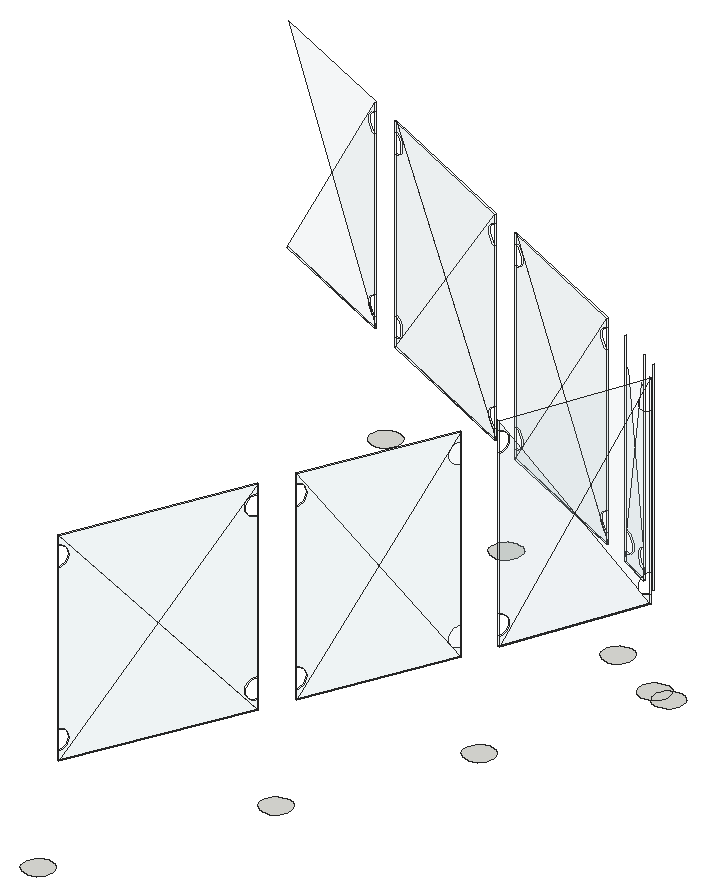
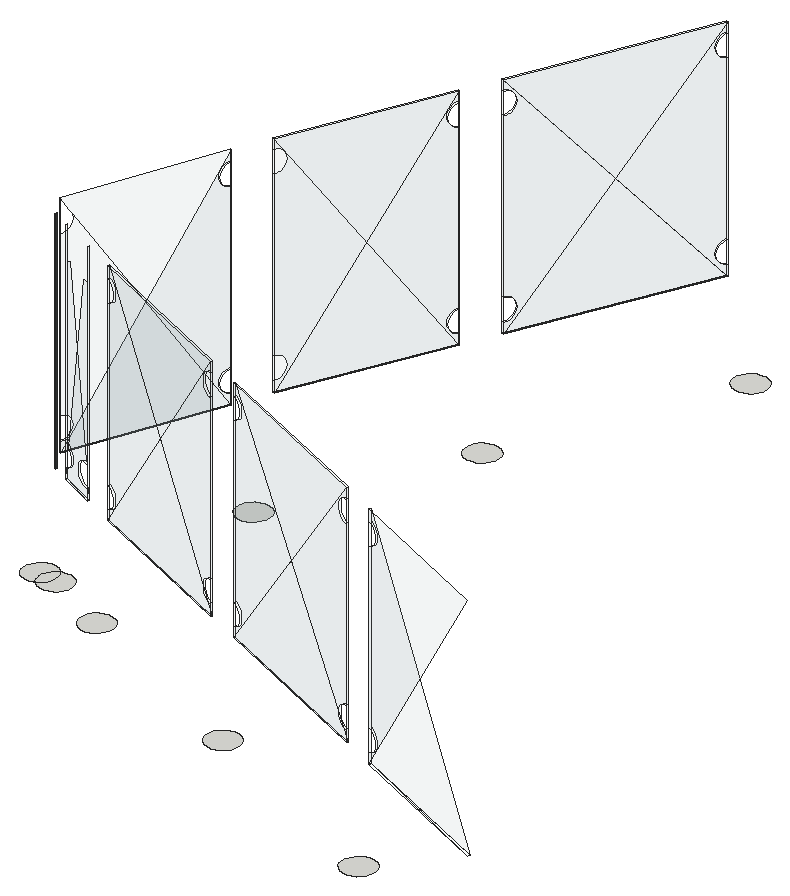
# SketchUp Ruby script. Lengths in inches.
U = 1.inch
M = Sketchup.active_model
def pt(a) = Geom::Point3d.new(a.map { |v| v * U })
def face(e, loops, mat)
  f = e.add_face(loops[0].map { |a| pt(a) })
  loops[1..].each { |l| e.add_face(l.map { |a| pt(a) }).erase! }
  f.material = f.back_material = mat if mat
  f
end
# faces: each face lists its corners as indices into pts; further lists are holes
def faces(e, pts, list, mat = nil) = list.each { |f| face(e, (f[0].is_a?(Array) ? f : [f]).map { |l| l.map { |i| pts[i] } }, mat) }
# xy, xz, yz: faces in a plane at the given z, y or x. An outline is a flat list of corners, or four numbers for a rectangle; further outlines are holes
def ring(l) = l.size == 4 ? [[l[0], l[1]], [l[2], l[1]], [l[2], l[3]], [l[0], l[3]]] : l.each_slice(2).to_a
def flat(e, list, mat, &to3) = list.each { |f| face(e, (f[0].is_a?(Array) ? f : [f]).map { |l| ring(l).map { |u, v| to3.(u, v) } }, mat) }
def xy(e, z, list, mat = nil) = flat(e, list, mat) { |x, y| [x, y, z] }
def xz(e, y, list, mat = nil) = flat(e, list, mat) { |x, z| [x, y, z] }
def yz(e, x, list, mat = nil) = flat(e, list, mat) { |y, z| [x, y, z] }
def lines(e, pts, list) = list.each { |a, b| e.add_line(pt(pts[a]), pt(pts[b])) }
# prism: a flat outline (further loops are holes) pulled along v
def prism(e, loops, v, mat = nil)
  f = face(e, loops, mat); d = Geom::Vector3d.new(v.map { |x| x * U })
  f.pushpull(f.normal.samedirection?(d) ? d.length : -d.length)
end
def box(e, o, s, mat = nil) = prism(e, [[o, [o[0] + s[0], o[1], o[2]], [o[0] + s[0], o[1] + s[1], o[2]], [o[0], o[1] + s[1], o[2]]]], [0, 0, s[2]], mat)
def at(x, y, z, deg = 0) = Geom::Transformation.translation(pt([x, y, z])) * Geom::Transformation.rotation(ORIGIN, Z_AXIS, deg.degrees)
def axes(o, x, y, z) = Geom::Transformation.new([*x, 0, *y, 0, *z, 0, *pt(o).to_a, 1])
def part(name) = M.definitions.add(name)
# library, detail: a bought-in or finely detailed component or shape, given as its bounding box
def library(name, o, s) = part(name).tap { |d| box(d.entities, o, s) }
def detail(e, o, s) = box(e.add_group.entities, o, s)
def put(e, d, t, mat = nil) = e.add_instance(d, t).tap { |i| i.material = mat if mat }
def group(e, t, mat = nil) = e.add_group.tap { |g| g.transformation = t; g.material = mat if mat }.entities
root = M.entities
M.materials.add("Glass_Safety_01").color = [204, 235, 244]
M.materials["Glass_Safety_01"].alpha = 0.1
xy(root,321.858,[[999.761,953.602,1000.164,953.685,1000.532,953.869,1000.839,954.142,1001.065,954.485,1001.195,954.875,1001.219,955.286,1001.137,955.688,1000.953,956.056,1000.68,956.363,1000.337,956.59,999.946,956.719,999.536,956.744,999.133,956.661,998.766,956.477,998.458,956.204,998.232,955.861,998.102,955.471,998.078,955.06,998.161,954.658,998.345,954.29,998.618,953.983,998.961,953.756,999.351,953.627],[1009.107,975.06,1009.51,975.143,1009.877,975.327,1010.185,975.6,1010.411,975.943,1010.541,976.333,1010.565,976.744,1010.482,977.146,1010.298,977.514,1010.025,977.821,1009.682,978.048,1009.292,978.177,1008.882,978.202,1008.479,978.119,1008.111,977.935,1007.804,977.662,1007.578,977.319,1007.448,976.929,1007.423,976.518,1007.506,976.116,1007.69,975.748,1007.963,975.441,1008.306,975.214,1008.696,975.085],[1017.079,993.365,1017.482,993.447,1017.849,993.631,1018.157,993.904,1018.383,994.248,1018.513,994.638,1018.537,995.048,1018.455,995.451,1018.27,995.818,1017.998,996.126,1017.654,996.352,1017.264,996.482,1016.854,996.506,1016.451,996.424,1016.084,996.24,1015.776,995.967,1015.55,995.623,1015.42,995.233,1015.396,994.823,1015.478,994.42,1015.662,994.053,1015.935,993.745,1016.279,993.519,1016.669,993.389],[1023.991,1011.073,1024.394,1011.156,1024.762,1011.34,1025.069,1011.613,1025.295,1011.956,1025.425,1012.346,1025.45,1012.756,1025.367,1013.159,1025.183,1013.527,1024.91,1013.834,1024.567,1014.061,1024.177,1014.19,1023.766,1014.215,1023.363,1014.132,1023.238,1014.069,1023.367,1013.924,1023.551,1013.556,1023.634,1013.153,1023.609,1012.743,1023.48,1012.353,1023.253,1012.01,1022.946,1011.737,1022.704,1011.616,1022.848,1011.454,1023.191,1011.227,1023.581,1011.098],[1022.175,1011.47,1022.578,1011.553,1022.704,1011.616,1022.575,1011.761,1022.391,1012.129,1022.308,1012.531,1022.332,1012.942,1022.462,1013.332,1022.688,1013.675,1022.996,1013.948,1023.238,1014.069,1023.094,1014.231,1022.751,1014.457,1022.361,1014.587,1021.95,1014.611,1021.548,1014.529,1021.18,1014.345,1020.873,1014.072,1020.646,1013.729,1020.516,1013.338,1020.492,1012.928,1020.575,1012.525,1020.759,1012.158,1021.032,1011.85,1021.375,1011.624,1021.765,1011.494],
  [1022.704,1011.616,1022.946,1011.737,1023.253,1012.01,1023.48,1012.353,1023.609,1012.743,1023.634,1013.153,1023.551,1013.556,1023.367,1013.924,1023.238,1014.069,1022.996,1013.948,1022.688,1013.675,1022.462,1013.332,1022.332,1012.942,1022.308,1012.531,1022.391,1012.129,1022.575,1011.761],[1015.608,1014.567,1016.011,1014.65,1016.378,1014.834,1016.686,1015.107,1016.912,1015.45,1017.042,1015.84,1017.066,1016.251,1016.983,1016.653,1016.799,1017.021,1016.526,1017.328,1016.183,1017.555,1015.793,1017.684,1015.383,1017.709,1014.98,1017.626,1014.612,1017.442,1014.305,1017.169,1014.079,1016.826,1013.949,1016.436,1013.924,1016.025,1014.007,1015.623,1014.191,1015.255,1014.464,1014.948,1014.807,1014.721,1015.197,1014.592],[996.475,1022.9,996.878,1022.983,997.246,1023.167,997.553,1023.44,997.779,1023.783,997.909,1024.173,997.934,1024.583,997.851,1024.986,997.667,1025.354,997.394,1025.661,997.051,1025.887,996.661,1026.017,996.25,1026.042,995.848,1025.959,995.48,1025.775,995.172,1025.502,994.946,1025.159,994.816,1024.769,994.792,1024.358,994.875,1023.955,995.059,1023.588,995.332,1023.28,995.675,1023.054,996.065,1022.924],[975.893,1031.864,976.296,1031.947,976.663,1032.131,976.971,1032.404,977.197,1032.747,977.327,1033.137,977.351,1033.548,977.269,1033.95,977.085,1034.318,976.812,1034.625,976.468,1034.852,976.078,1034.981,975.668,1035.006,975.265,1034.923,974.898,1034.739,974.59,1034.466,974.364,1034.123,974.234,1033.733,974.21,1033.322,974.292,1032.92,974.476,1032.552,974.749,1032.245,975.093,1032.018,975.483,1031.889]])
xy(root,331.897,[[1000.525,956.939,1000.344,957.017,1008.365,974.939],[1000.344,957.017,1008.184,975.017,1008.365,974.939],[1009.871,978.396,1009.69,978.475,1016.348,993.269],[1009.69,978.475,1016.168,993.348,1016.348,993.269],[1017.774,996.733,1017.591,996.805,1023.329,1010.964],
  [1017.591,996.805,1023.145,1011.036,1023.329,1010.964],[1021.935,1012.968,1021.928,1012.969,1021.97,1013.162],[1021.935,1012.968,1021.97,1013.162,1021.977,1013.16],[1020.24,1013.791,1016.751,1015.437,1016.835,1015.615],[1020.24,1013.791,1016.835,1015.615,1020.324,1013.969],
  [1013.651,1016.834,997.958,1023.669,998.037,1023.849],[1013.651,1016.834,998.037,1023.849,1013.73,1017.014],[994.519,1025.167,977.388,1032.628,977.466,1032.808],[994.519,1025.167,977.466,1032.808,994.597,1025.347],[973.936,1034.131,958.914,1040.674,958.992,1040.854],
  [973.936,1034.131,958.992,1040.854,974.015,1034.311]],"Glass_Safety_01")
p = [[1000.344,957.017,331.897],[1000.525,956.939,331.897],[1000.525,956.939,333],[1000.525,956.939,335.125],[1000.525,956.939,351.283],[1000.525,956.939,353.409],
  [1000.525,956.939,354.511],[1000.344,957.017,354.511],[1000.344,957.017,353.409],[1000.344,957.017,351.283],[1000.344,957.017,335.125],[1000.344,957.017,333],
  [1000.635,957.191,335.089],[1000.737,957.426,334.983],[1000.825,957.628,334.814],[1000.893,957.783,334.594],[1000.935,957.88,334.338],[1000.949,957.913,334.0625],
  [1000.935,957.88,333.787],[1000.893,957.783,333.531],[1000.825,957.628,333.311],[1000.737,957.426,333.142],[1000.635,957.191,333.036],[1008.365,974.939,354.511],
  [1000.635,957.191,353.373],[1000.737,957.426,353.267],[1000.825,957.628,353.098],[1000.893,957.783,352.877],[1000.935,957.88,352.621],[1000.949,957.913,352.346],
  [1000.935,957.88,352.071],[1000.893,957.783,351.814],[1000.825,957.628,351.594],[1000.737,957.426,351.425],[1000.635,957.191,351.319],[1008.365,974.939,331.897],
  [1008.365,974.939,333],[1008.298,974.787,333],[1008.189,974.535,333.036],[1008.086,974.3,333.142],[1007.998,974.098,333.311],[1007.931,973.943,333.531],
  [1007.888,973.846,333.787],[1007.874,973.8125,334.0625],[1007.888,973.846,334.338],[1007.931,973.943,334.594],[1007.998,974.098,334.814],[1008.086,974.3,334.983],
  [1008.189,974.535,335.089],[1008.298,974.787,335.125],[1008.365,974.939,335.125],[1008.365,974.939,351.283],[1008.298,974.787,351.283],[1008.189,974.535,351.319],
  [1008.086,974.3,351.425],[1007.998,974.098,351.594],[1007.931,973.943,351.814],[1007.888,973.846,352.071],[1007.874,973.8125,352.346],[1007.888,973.846,352.621],
  [1007.931,973.943,352.877],[1007.998,974.098,353.098],[1008.086,974.3,353.267],[1008.189,974.535,353.373],[1008.298,974.787,353.409],[1008.365,974.939,353.409],
  [1000.454,957.269,333.036],[1000.557,957.504,333.142],[1000.645,957.706,333.311],[1000.712,957.861,333.531],[1000.754,957.958,333.787],[1000.769,957.992,334.0625],
  [1000.754,957.958,334.338],[1000.712,957.861,334.594],[1000.645,957.706,334.814],[1000.557,957.504,334.983],[1000.454,957.269,335.089],[1000.454,957.269,351.319],
  [1000.557,957.504,351.425],[1000.645,957.706,351.594],[1000.712,957.861,351.814],[1000.754,957.958,352.071],[1000.769,957.992,352.346],[1000.754,957.958,352.621],
  [1000.712,957.861,352.877],[1000.645,957.706,353.098],[1000.557,957.504,353.267],[1000.454,957.269,353.373],[1008.184,975.017,331.897],[1008.184,975.017,351.283],
  [1008.184,975.017,335.125],[1008.118,974.865,335.125],[1008.008,974.613,335.089],[1007.906,974.378,334.983],[1007.818,974.176,334.814],[1007.75,974.021,334.594],
  [1007.708,973.924,334.338],[1007.694,973.891,334.0625],[1007.708,973.924,333.787],[1007.75,974.021,333.531],[1007.818,974.176,333.311],[1007.906,974.378,333.142],
  [1008.008,974.613,333.036],[1008.118,974.865,333],[1008.184,975.017,333],[1008.184,975.017,354.511],[1008.184,975.017,353.409],[1008.118,974.865,353.409],
  [1008.008,974.613,353.373],[1007.906,974.378,353.267],[1007.818,974.176,353.098],[1007.75,974.021,352.877],[1007.708,973.924,352.621],[1007.694,973.891,352.346],
  [1007.708,973.924,352.071],[1007.75,974.021,351.814],[1007.818,974.176,351.594],[1007.906,974.378,351.425],[1008.008,974.613,351.319],[1008.118,974.865,351.283],
  [1009.69,978.475,331.897],[1009.871,978.396,331.897],[1009.871,978.396,333],[1009.871,978.396,335.125],[1009.871,978.396,351.283],[1009.871,978.396,353.409],
  [1009.871,978.396,354.511],[1009.69,978.475,354.511],[1009.69,978.475,353.409],[1009.69,978.475,351.283],[1009.69,978.475,335.125],[1009.69,978.475,333],
  [1009.98,978.649,335.089],[1010.083,978.884,334.983],[1010.171,979.086,334.814],[1010.238,979.24,334.594],[1010.28,979.338,334.338],[1010.295,979.371,334.0625],
  [1010.28,979.338,333.787],[1010.238,979.24,333.531],[1010.171,979.086,333.311],[1010.083,978.884,333.142],[1009.98,978.649,333.036],[1016.348,993.269,354.511],
  [1009.98,978.649,353.373],[1010.083,978.884,353.267],[1010.171,979.086,353.098],[1010.238,979.24,352.877],[1010.28,979.338,352.621],[1010.295,979.371,352.346],
  [1010.28,979.338,352.071],[1010.238,979.24,351.814],[1010.171,979.086,351.594],[1010.083,978.884,351.425],[1009.98,978.649,351.319],[1016.348,993.269,331.897],
  [1016.348,993.269,333],[1016.271,993.091,333],[1016.161,992.839,333.036],[1016.058,992.604,333.142],[1015.97,992.402,333.311],[1015.903,992.247,333.531],
  [1015.861,992.15,333.787],[1015.846,992.117,334.0625],[1015.861,992.15,334.338],[1015.903,992.247,334.594],[1015.97,992.402,334.814],[1016.058,992.604,334.983],
  [1016.161,992.839,335.089],[1016.271,993.091,335.125],[1016.348,993.269,335.125],[1016.348,993.269,351.283],[1016.271,993.091,351.283],[1016.161,992.839,351.319],
  [1016.058,992.604,351.425],[1015.97,992.402,351.594],[1015.903,992.247,351.814],[1015.861,992.15,352.071],[1015.846,992.117,352.346],[1015.861,992.15,352.621],
  [1015.903,992.247,352.877],[1015.97,992.402,353.098],[1016.058,992.604,353.267],[1016.161,992.839,353.373],[1016.271,993.091,353.409],[1016.348,993.269,353.409],
  [1009.8,978.727,333.036],[1009.902,978.962,333.142],[1009.99,979.164,333.311],[1010.058,979.319,333.531],[1010.1,979.416,333.787],[1010.114,979.45,334.0625],
  [1010.1,979.416,334.338],[1010.058,979.319,334.594],[1009.99,979.164,334.814],[1009.902,978.962,334.983],[1009.8,978.727,335.089],[1009.8,978.727,351.319],
  [1009.902,978.962,351.425],[1009.99,979.164,351.594],[1010.058,979.319,351.814],[1010.1,979.416,352.071],[1010.114,979.45,352.346],[1010.1,979.416,352.621],
  [1010.058,979.319,352.877],[1009.99,979.164,353.098],[1009.902,978.962,353.267],[1009.8,978.727,353.373],[1016.168,993.348,331.897],[1016.168,993.348,354.511],
  [1016.168,993.348,353.409],[1016.168,993.348,351.283],[1016.168,993.348,335.125],[1016.168,993.348,333],[1017.591,996.805,331.897],[1017.774,996.733,331.897],
  [1017.774,996.733,333],[1017.774,996.733,335.125],[1017.774,996.733,351.283],[1017.774,996.733,353.409],[1017.774,996.733,354.511],[1017.591,996.805,354.511],
  [1017.591,996.805,353.409],[1017.591,996.805,351.283],[1017.591,996.805,335.125],[1017.591,996.805,333],[1017.874,996.99,335.089],[1017.967,997.229,334.983],
  [1018.047,997.434,334.814],[1018.109,997.591,334.594],[1018.147,997.69,334.338],[1018.16,997.724,334.0625],[1018.147,997.69,333.787],[1018.109,997.591,333.531],
  [1018.047,997.434,333.311],[1017.967,997.229,333.142],[1017.874,996.99,333.036],[1022.908,1009.886,352.798],[1022.92,1009.917,352.877],[1022.981,1010.074,353.098],
  [1022.982,1010.075,353.098],[1023.329,1010.964,354.511],[1017.874,996.99,353.373],[1017.967,997.229,353.267],[1018.047,997.434,353.098],[1018.109,997.591,352.877],
  [1018.147,997.69,352.621],[1018.16,997.724,352.346],[1018.147,997.69,352.071],[1018.109,997.591,351.814],[1018.047,997.434,351.594],[1017.967,997.229,351.425],
  [1017.874,996.99,351.319],[1023.329,1010.964,335.125],[1023.329,1010.964,351.283],[1023.255,1010.774,351.283],[1023.155,1010.518,351.319],[1023.061,1010.279,351.425],
  [1022.981,1010.074,351.594],[1022.92,1009.917,351.814],[1022.881,1009.818,352.071],[1022.868,1009.784,352.346],[1022.881,1009.818,352.621],[1023.329,1010.964,331.897],
  [1023.329,1010.964,333],[1023.255,1010.774,333],[1023.155,1010.518,333.036],[1023.061,1010.279,333.142],[1022.981,1010.074,333.311],[1022.92,1009.917,333.531],
  [1022.881,1009.818,333.787],[1022.868,1009.784,334.0625],[1022.881,1009.818,334.338],[1022.92,1009.917,334.594],[1022.981,1010.074,334.814],[1023.061,1010.279,334.983],
  [1023.155,1010.518,335.089],[1023.255,1010.774,335.125],[1017.691,997.061,351.319],[1017.784,997.3,351.425],[1017.864,997.505,351.594],[1017.925,997.663,351.814],
  [1017.964,997.762,352.071],[1017.977,997.795,352.346],[1017.964,997.762,352.621],[1017.925,997.663,352.877],[1017.864,997.505,353.098],[1017.784,997.3,353.267],
  [1017.691,997.061,353.373],[1022.725,1009.958,333.61],[1022.737,1009.988,333.531],[1022.798,1010.146,333.311],[1022.798,1010.147,333.31],[1023.145,1011.036,331.897],
  [1017.691,997.061,333.036],[1017.784,997.3,333.142],[1017.864,997.505,333.311],[1017.925,997.663,333.531],[1017.964,997.762,333.787],[1017.977,997.795,334.0625],
  [1017.964,997.762,334.338],[1017.925,997.663,334.594],[1017.864,997.505,334.814],[1017.784,997.3,334.983],[1017.691,997.061,335.089],[1022.878,1010.351,333.142],
  [1022.971,1010.59,333.036],[1023.071,1010.846,333],[1023.145,1011.036,333],[1023.145,1011.036,335.125],[1023.145,1011.036,351.283],[1023.145,1011.036,353.409],
  [1023.145,1011.036,354.511],[1023.329,1010.964,353.409],[1021.935,1012.968,331.897],[1021.935,1012.968,333],[1021.929,1012.969,333],[1021.928,1012.969,331.897],
  [1021.977,1013.16,331.897],[1021.977,1013.16,333],[1021.977,1013.16,335.125],[1021.977,1013.16,351.283],[1021.977,1013.16,353.409],[1021.977,1013.16,354.511],
  [1021.935,1012.968,354.511],[1021.935,1012.968,353.409],[1021.935,1012.968,351.283],[1021.935,1012.968,335.125],[1021.97,1013.162,331.897],[1021.929,1012.969,335.125],
  [1021.928,1012.969,351.284],[1021.928,1012.969,353.408],[1021.928,1012.969,354.511],[1021.97,1013.162,354.511],[1021.971,1013.162,353.408],[1021.971,1013.161,351.284],
  [1021.97,1013.162,335.125],[1021.97,1013.162,333],[1019.764,1014.016,351.423],[1017.249,1015.202,335.123],[1017.483,1015.092,335.089],[1017.714,1014.983,334.983],
  [1017.914,1014.889,334.814],[1018.066,1014.817,334.594],[1018.162,1014.771,334.338],[1018.195,1014.756,334.0625],[1018.162,1014.771,333.787],[1018.066,1014.817,333.531],
  [1017.914,1014.889,333.311],[1017.714,1014.983,333.142],[1017.483,1015.092,333.036],[1017.234,1015.209,333],[1016.921,1015.357,333],[1016.751,1015.437,331.897],
  [1020.24,1013.791,331.897],[1020.24,1013.791,333],[1019.992,1013.909,333.036],[1019.76,1014.018,333.142],[1019.561,1014.112,333.311],[1019.408,1014.184,333.531],
  [1019.312,1014.229,333.787],[1019.279,1014.245,334.0625],[1019.312,1014.229,334.338],[1019.408,1014.184,334.594],[1019.561,1014.112,334.814],[1019.76,1014.018,334.983],
  [1019.992,1013.909,335.089],[1020.24,1013.791,335.125],[1020.24,1013.791,351.283],[1019.992,1013.909,351.319],[1020.324,1013.969,331.897],[1020.324,1013.969,333],
  [1020.324,1013.969,335.125],[1020.324,1013.969,351.283],[1020.324,1013.969,353.409],[1020.324,1013.969,354.511],[1020.24,1013.791,354.511],[1020.24,1013.791,353.409],
  [1017.333,1015.38,351.285],[1019.848,1014.194,334.985],[1019.844,1014.196,334.983],[1019.645,1014.29,334.814],[1019.492,1014.362,334.594],[1019.396,1014.407,334.338],
  [1019.363,1014.423,334.0625],[1019.396,1014.407,333.787],[1019.492,1014.362,333.531],[1019.645,1014.29,333.311],[1019.844,1014.196,333.142],[1020.076,1014.087,333.036],
  [1020.15,1014.051,333.025],[1016.835,1015.615,331.897],[1016.835,1015.615,333],[1017.318,1015.387,333],[1017.567,1015.27,333.036],[1017.798,1015.161,333.142],
  [1017.998,1015.067,333.311],[1018.15,1014.995,333.531],[1018.246,1014.949,333.787],[1018.279,1014.934,334.0625],[1018.246,1014.949,334.338],[1018.15,1014.995,334.594],
  [1017.998,1015.067,334.814],[1017.798,1015.161,334.983],[1017.567,1015.27,335.089],[1017.318,1015.387,335.125],[1016.835,1015.615,335.125],[1016.835,1015.615,351.283],
  [1017.318,1015.387,351.283],[1016.751,1015.437,333],[1016.751,1015.437,333.078],[1016.751,1015.437,335.047],[1016.751,1015.437,335.125],[1016.751,1015.437,351.283],
  [1016.751,1015.437,351.362],[1016.751,1015.437,353.33],[1016.751,1015.437,353.409],[1016.751,1015.437,354.511],[1016.835,1015.615,354.511],[1016.835,1015.615,353.409],
  [1016.835,1015.615,353.33],[1016.835,1015.615,351.362],[1016.835,1015.615,335.047],[1016.835,1015.615,333.078],[1013.651,1016.834,331.897],[1013.651,1016.834,333],
  [1013.399,1016.944,333.036],[1013.164,1017.046,333.142],[1012.962,1017.134,333.311],[1012.807,1017.201,333.531],[1012.71,1017.244,333.787],[1012.677,1017.258,334.0625],
  [1012.71,1017.244,334.338],[1012.807,1017.201,334.594],[1012.962,1017.134,334.814],[1013.164,1017.046,334.983],[1013.399,1016.944,335.089],[1013.651,1016.834,335.125],
  [1013.651,1016.834,351.283],[1013.399,1016.944,351.319],[1013.164,1017.046,351.425],[1012.962,1017.134,351.594],[1012.807,1017.201,351.814],[1012.71,1017.244,352.071],
  [1012.677,1017.258,352.346],[1012.71,1017.244,352.621],[1012.807,1017.201,352.877],[1012.962,1017.134,353.098],[1013.164,1017.046,353.267],[1013.399,1016.944,353.373],
  [1013.651,1016.834,353.409],[1013.651,1016.834,354.511],[997.958,1023.669,331.897],[997.958,1023.669,351.283],[997.958,1023.669,335.125],[998.128,1023.594,335.125],
  [998.381,1023.485,335.089],[998.616,1023.382,334.983],[998.817,1023.294,334.814],[998.972,1023.227,334.594],[999.07,1023.184,334.338],[999.103,1023.17,334.0625],
  [999.07,1023.184,333.787],[998.972,1023.227,333.531],[998.817,1023.294,333.311],[998.616,1023.382,333.142],[998.381,1023.485,333.036],[998.128,1023.594,333],
  [997.958,1023.669,333],[997.958,1023.669,354.511],[997.958,1023.669,353.409],[998.128,1023.594,353.409],[998.381,1023.485,353.373],[998.616,1023.382,353.267],
  [998.817,1023.294,353.098],[998.972,1023.227,352.877],[999.07,1023.184,352.621],[999.103,1023.17,352.346],[999.07,1023.184,352.071],[998.972,1023.227,351.814],
  [998.817,1023.294,351.594],[998.616,1023.382,351.425],[998.381,1023.485,351.319],[998.128,1023.594,351.283],[1013.73,1017.014,331.897],[1013.73,1017.014,333],
  [1013.73,1017.014,335.125],[1013.73,1017.014,351.283],[1013.73,1017.014,353.409],[1013.73,1017.014,354.511],[1013.478,1017.124,335.089],[1013.242,1017.226,334.983],
  [1013.041,1017.314,334.814],[1012.886,1017.382,334.594],[1012.788,1017.424,334.338],[1012.755,1017.439,334.0625],[1012.788,1017.424,333.787],[1012.886,1017.382,333.531],
  [1013.041,1017.314,333.311],[1013.242,1017.226,333.142],[1013.478,1017.124,333.036],[998.037,1023.849,354.511],[1013.478,1017.124,353.373],[1013.242,1017.226,353.267],
  [1013.041,1017.314,353.098],[1012.886,1017.382,352.877],[1012.788,1017.424,352.621],[1012.755,1017.439,352.346],[1012.788,1017.424,352.071],[1012.886,1017.382,351.814],
  [1013.041,1017.314,351.594],[1013.242,1017.226,351.425],[1013.478,1017.124,351.319],[998.037,1023.849,331.897],[998.037,1023.849,333],[998.207,1023.775,333],
  [998.459,1023.665,333.036],[998.694,1023.563,333.142],[998.896,1023.475,333.311],[999.051,1023.407,333.531],[999.148,1023.365,333.787],[999.181,1023.35,334.0625],
  [999.148,1023.365,334.338],[999.051,1023.407,334.594],[998.896,1023.475,334.814],[998.694,1023.563,334.983],[998.459,1023.665,335.089],[998.207,1023.775,335.125],
  [998.037,1023.849,335.125],[998.037,1023.849,351.283],[998.207,1023.775,351.283],[998.459,1023.665,351.319],[998.694,1023.563,351.425],[998.896,1023.475,351.594],
  [999.051,1023.407,351.814],[999.148,1023.365,352.071],[999.181,1023.35,352.346],[999.148,1023.365,352.621],[999.051,1023.407,352.877],[998.896,1023.475,353.098],
  [998.694,1023.563,353.267],[998.459,1023.665,353.373],[998.207,1023.775,353.409],[998.037,1023.849,353.409],[994.519,1025.167,331.897],[994.519,1025.167,333],
  [994.267,1025.276,333.036],[994.031,1025.379,333.142],[993.83,1025.467,333.311],[993.675,1025.534,333.531],[993.577,1025.577,333.787],[993.544,1025.591,334.0625],
  [993.577,1025.577,334.338],[993.675,1025.534,334.594],[993.83,1025.467,334.814],[994.031,1025.379,334.983],[994.267,1025.276,335.089],[994.519,1025.167,335.125],
  [994.519,1025.167,351.283],[994.267,1025.276,351.319],[994.031,1025.379,351.425],[993.83,1025.467,351.594],[993.675,1025.534,351.814],[993.577,1025.577,352.071],
  [993.544,1025.591,352.346],[993.577,1025.577,352.621],[993.675,1025.534,352.877],[993.83,1025.467,353.098],[994.031,1025.379,353.267],[994.267,1025.276,353.373],
  [994.519,1025.167,353.409],[994.519,1025.167,354.511],[977.388,1032.628,331.897],[977.388,1032.628,351.283],[977.388,1032.628,335.125],[977.546,1032.559,335.125],
  [977.798,1032.449,335.089],[978.033,1032.346,334.983],[978.235,1032.259,334.814],[978.39,1032.191,334.594],[978.487,1032.149,334.338],[978.521,1032.134,334.0625],
  [978.487,1032.149,333.787],[978.39,1032.191,333.531],[978.235,1032.259,333.311],[978.033,1032.346,333.142],[977.798,1032.449,333.036],[977.546,1032.559,333],
  [977.388,1032.628,333],[977.388,1032.628,354.511],[977.388,1032.628,353.409],[977.546,1032.559,353.409],[977.798,1032.449,353.373],[978.033,1032.346,353.267],
  [978.235,1032.259,353.098],[978.39,1032.191,352.877],[978.487,1032.149,352.621],[978.521,1032.134,352.346],[978.487,1032.149,352.071],[978.39,1032.191,351.814],
  [978.235,1032.259,351.594],[978.033,1032.346,351.425],[977.798,1032.449,351.319],[977.546,1032.559,351.283],[994.597,1025.347,331.897],[994.597,1025.347,333],
  [994.597,1025.347,335.125],[994.597,1025.347,351.283],[994.597,1025.347,353.409],[994.597,1025.347,354.511],[994.345,1025.457,335.089],[994.11,1025.559,334.983],
  [993.908,1025.647,334.814],[993.753,1025.715,334.594],[993.656,1025.757,334.338],[993.623,1025.771,334.0625],[993.656,1025.757,333.787],[993.753,1025.715,333.531],
  [993.908,1025.647,333.311],[994.11,1025.559,333.142],[994.345,1025.457,333.036],[977.466,1032.808,354.511],[994.345,1025.457,353.373],[994.11,1025.559,353.267],
  [993.908,1025.647,353.098],[993.753,1025.715,352.877],[993.656,1025.757,352.621],[993.623,1025.771,352.346],[993.656,1025.757,352.071],[993.753,1025.715,351.814],
  [993.908,1025.647,351.594],[994.11,1025.559,351.425],[994.345,1025.457,351.319],[977.466,1032.808,331.897],[977.466,1032.808,333],[977.625,1032.739,333],
  [977.877,1032.629,333.036],[978.112,1032.527,333.142],[978.314,1032.439,333.311],[978.469,1032.372,333.531],[978.566,1032.329,333.787],[978.599,1032.315,334.0625],
  [978.566,1032.329,334.338],[978.469,1032.372,334.594],[978.314,1032.439,334.814],[978.112,1032.527,334.983],[977.877,1032.629,335.089],[977.625,1032.739,335.125],
  [977.466,1032.808,335.125],[977.466,1032.808,351.283],[977.625,1032.739,351.283],[977.877,1032.629,351.319],[978.112,1032.527,351.425],[978.314,1032.439,351.594],
  [978.469,1032.372,351.814],[978.566,1032.329,352.071],[978.599,1032.315,352.346],[978.566,1032.329,352.621],[978.469,1032.372,352.877],[978.314,1032.439,353.098],
  [978.112,1032.527,353.267],[977.877,1032.629,353.373],[977.625,1032.739,353.409],[977.466,1032.808,353.409],[973.936,1034.131,331.897],[973.936,1034.131,333],
  [973.684,1034.241,333.036],[973.449,1034.343,333.142],[973.247,1034.431,333.311],[973.092,1034.498,333.531],[972.995,1034.541,333.787],[972.962,1034.555,334.0625],
  [972.995,1034.541,334.338],[973.092,1034.498,334.594],[973.247,1034.431,334.814],[973.449,1034.343,334.983],[973.684,1034.241,335.089],[973.936,1034.131,335.125],
  [973.936,1034.131,351.283],[973.684,1034.241,351.319],[973.449,1034.343,351.425],[973.247,1034.431,351.594],[973.092,1034.498,351.814],[972.995,1034.541,352.071],
  [972.962,1034.555,352.346],[972.995,1034.541,352.621],[973.092,1034.498,352.877],[973.247,1034.431,353.098],[973.449,1034.343,353.267],[973.684,1034.241,353.373],
  [973.936,1034.131,353.409],[973.936,1034.131,354.511],[958.914,1040.674,331.897],[974.015,1034.311,331.897],[974.015,1034.311,333],[974.015,1034.311,335.125],
  [974.015,1034.311,351.283],[974.015,1034.311,353.409],[974.015,1034.311,354.511],[973.763,1034.421,335.089],[973.528,1034.523,334.983],[973.326,1034.611,334.814],
  [973.171,1034.679,334.594],[973.074,1034.721,334.338],[973.04,1034.736,334.0625],[973.074,1034.721,333.787],[973.171,1034.679,333.531],[973.326,1034.611,333.311],
  [973.528,1034.523,333.142],[973.763,1034.421,333.036],[958.992,1040.854,354.511],[973.763,1034.421,353.373],[973.528,1034.523,353.267],[973.326,1034.611,353.098],
  [973.171,1034.679,352.877],[973.074,1034.721,352.621],[973.04,1034.736,352.346],[973.074,1034.721,352.071],[973.171,1034.679,351.814],[973.326,1034.611,351.594],
  [973.528,1034.523,351.425],[973.763,1034.421,351.319]]
faces(root,p,[[0,1,2,3,4,5,6,7,8,9,10,11],[4,3,12,13,14,15,16,17,18,19,20,21,22,2,1,23,6,5,24,25,26,27,28,29,30,31,32,33,34],[35,36,37,38,39,40,41,42,43,44,45,46,47,48,49,50,51,52,53,54,55,56,57,58,59,60,61,62,63,64,65,23,1],[0,11,66,67,68,69,70,71,72,73,74,75,76,10,9,77,78,79,80,81,82,83,84,85,86,87,8,7,88],[89,90,91,92,93,94,95,96,97,98,99,100,101,102,103,104,88,7,105,106,107,108,109,110,111,112,113,114,115,116,117,118,119],[35,88,104,90,89,106,105,23,65,51,50,36],[120,121,122,123,124,125,126,127,128,129,130,131],[124,123,132,133,134,135,136,137,138,139,140,141,142,122,121,143,126,125,144,145,146,147,148,149,150,151,152,153,154],
  [155,156,157,158,159,160,161,162,163,164,165,166,167,168,169,170,171,172,173,174,175,176,177,178,179,180,181,182,183,184,185,143,121],[120,131,186,187,188,189,190,191,192,193,194,195,196,130,129,197,198,199,200,201,202,203,204,205,206,207,128,127,208],[208,127,209,210,211,212,213],[155,208,213,212,211,210,209,143,185,171,170,156],[214,215,216,217,218,219,220,221,222,223,224,225],[218,217,226,227,228,229,230,231,232,233,234,235,236,216,215,237,238,239,240,241,220,219,242,243,244,245,246,247,248,249,250,251,252],[253,254,255,256,257,258,259,260,261,262,237,215,263,264,265,266,267,268,269,270,271,272,273,274,275,276,277],[224,223,278,279,280,281,282,283,284,285,286,287,288,222,221,289,290,291,292,293,214,225,294,295,296,297,298,299,300,301,302,303,304],
  [293,292,305,306,307,308],[263,293,308,309,310,311,312,241,313,254,253,264],[314,315,316,317],[314,318,319,320,321,322,323,324,325,326,327,315],[328,317,316,329,330,331,332,333,334,335,336,337],[328,337,319,318],[338,339,340,341,342,343,344,345,346,347,348,349,350,351,352,353,354,355,356,357,358,359,360,361,362,363,364,365,366,367,368,369],[354,370,371,372,373,374,375,376,377,368,367,355],
  [378,379,380,381,382,383,384,385,386,387,388,389,390,370,391,392,393,394,395,396,397,398,399,400,401,402,403,404,405,406,407,408],[370,390,371],[353,352,409],[391,353,409,410,411,412,413,414,415,416,417,418,419,420,421,407,406,422,423,392],[424,425,426,427,428,429,430,431,432,433,434,435,436,437,438,439,440,441,442,443,444,445,446,447,448,449,450,451,452],[453,454,455,456,457,458,459,460,461,462,463,464,465,466,467,468,452,451,469,470,471,472,473,474,475,476,477,478,479,480,481,482,483],[424,484,485,486,487,488,489,451,450,438,437,425],[487,486,490,491,492,493,494,495,496,497,498,499,500,485,484,501,489,488,502,503,504,505,506,507,508,509,510,511,512],
  [513,514,515,516,517,518,519,520,521,522,523,524,525,526,527,528,529,530,531,532,533,534,535,536,537,538,539,540,541,542,543,501,484],[513,452,468,454,453,470,469,501,543,529,528,514],[544,545,546,547,548,549,550,551,552,553,554,555,556,557,558,559,560,561,562,563,564,565,566,567,568,569,570,571,572],[573,574,575,576,577,578,579,580,581,582,583,584,585,586,587,588,572,571,589,590,591,592,593,594,595,596,597,598,599,600,601,602,603],[544,604,605,606,607,608,609,571,570,558,557,545],[607,606,610,611,612,613,614,615,616,617,618,619,620,605,604,621,609,608,622,623,624,625,626,627,628,629,630,631,632],[633,634,635,636,637,638,639,640,641,642,643,644,645,646,647,648,649,650,651,652,653,654,655,656,657,658,659,660,661,662,663,621,604],[633,572,588,574,573,590,589,621,663,649,648,634],
  [664,665,666,667,668,669,670,671,672,673,674,675,676,677,678,679,680,681,682,683,684,685,686,687,688,689,690,691,692],[664,693,694,695,696,697,698,691,690,678,677,665],[696,695,699,700,701,702,703,704,705,706,707,708,709,694,693,710,698,697,711,712,713,714,715,716,717,718,719,720,721]],"Glass_Safety_01")
